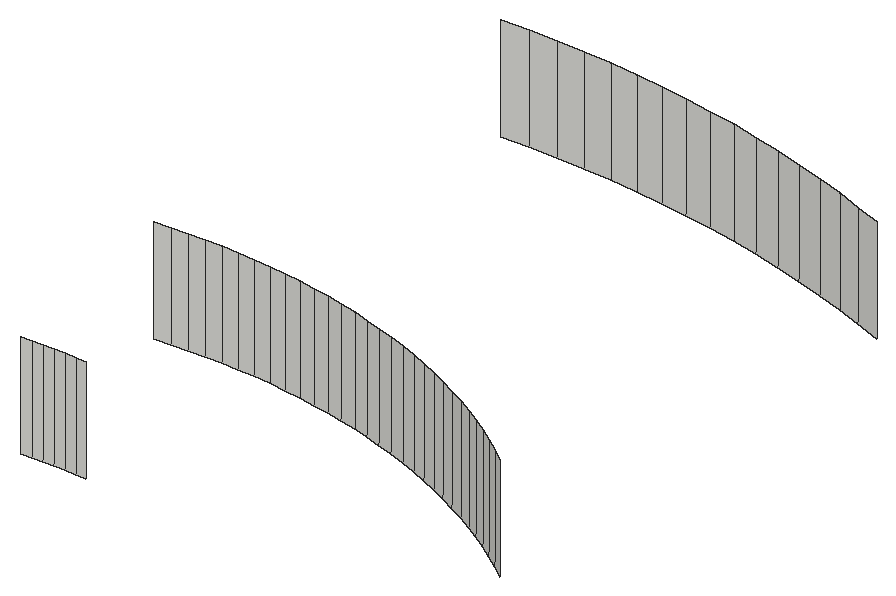
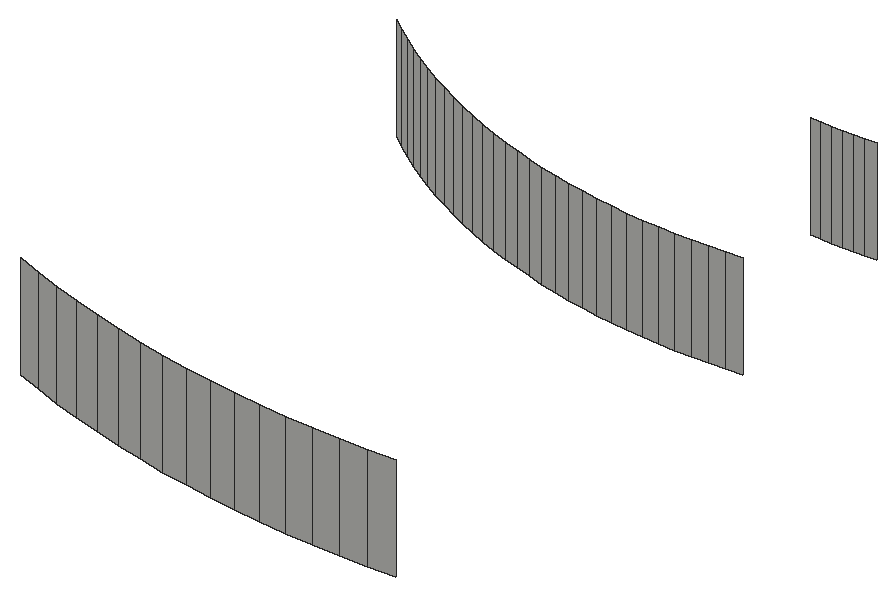
# SketchUp Ruby script. Lengths in inches.
U = 1.inch
M = Sketchup.active_model
def pt(a) = Geom::Point3d.new(a.map { |v| v * U })
def face(e, loops, mat)
  f = e.add_face(loops[0].map { |a| pt(a) })
  loops[1..].each { |l| e.add_face(l.map { |a| pt(a) }).erase! }
  f.material = f.back_material = mat if mat
  f
end
# faces: each face lists its corners as indices into pts; further lists are holes
def faces(e, pts, list, mat = nil) = list.each { |f| face(e, (f[0].is_a?(Array) ? f : [f]).map { |l| l.map { |i| pts[i] } }, mat) }
# xy, xz, yz: faces in a plane at the given z, y or x. An outline is a flat list of corners, or four numbers for a rectangle; further outlines are holes
def ring(l) = l.size == 4 ? [[l[0], l[1]], [l[2], l[1]], [l[2], l[3]], [l[0], l[3]]] : l.each_slice(2).to_a
def flat(e, list, mat, &to3) = list.each { |f| face(e, (f[0].is_a?(Array) ? f : [f]).map { |l| ring(l).map { |u, v| to3.(u, v) } }, mat) }
def xy(e, z, list, mat = nil) = flat(e, list, mat) { |x, y| [x, y, z] }
def xz(e, y, list, mat = nil) = flat(e, list, mat) { |x, z| [x, y, z] }
def yz(e, x, list, mat = nil) = flat(e, list, mat) { |y, z| [x, y, z] }
def lines(e, pts, list) = list.each { |a, b| e.add_line(pt(pts[a]), pt(pts[b])) }
# prism: a flat outline (further loops are holes) pulled along v
def prism(e, loops, v, mat = nil)
  f = face(e, loops, mat); d = Geom::Vector3d.new(v.map { |x| x * U })
  f.pushpull(f.normal.samedirection?(d) ? d.length : -d.length)
end
def box(e, o, s, mat = nil) = prism(e, [[o, [o[0] + s[0], o[1], o[2]], [o[0] + s[0], o[1] + s[1], o[2]], [o[0], o[1] + s[1], o[2]]]], [0, 0, s[2]], mat)
def at(x, y, z, deg = 0) = Geom::Transformation.translation(pt([x, y, z])) * Geom::Transformation.rotation(ORIGIN, Z_AXIS, deg.degrees)
def axes(o, x, y, z) = Geom::Transformation.new([*x, 0, *y, 0, *z, 0, *pt(o).to_a, 1])
def part(name) = M.definitions.add(name)
# library, detail: a bought-in or finely detailed component or shape, given as its bounding box
def library(name, o, s) = part(name).tap { |d| box(d.entities, o, s) }
def detail(e, o, s) = box(e.add_group.entities, o, s)
def put(e, d, t, mat = nil) = e.add_instance(d, t).tap { |i| i.material = mat if mat }
def group(e, t, mat = nil) = e.add_group.tap { |g| g.transformation = t; g.material = mat if mat }.entities
root = M.entities
p = [[904.72,349.22,117.3125],[904.1,349.18,117.3125],[904.1,349.18,111.3125],[904.72,349.22,111.3125],[905.35,349.25,117.3125],[905.35,349.25,111.3125],
  [905.98,349.26,117.3125],[905.98,349.26,111.3125],[906.61,349.25,117.3125],[906.61,349.25,111.3125],[907.23,349.22,117.3125],[907.23,349.22,111.3125],
  [907.86,349.18,117.3125],[907.86,349.18,111.3125],[927.14,354.38,117.3125],[927.89,353.82,117.3125],[927.89,353.82,111.3125],[927.14,354.38,111.3125],
  [926.37,354.92,117.3125],[926.37,354.92,111.3125],[925.59,355.45,117.3125],[925.59,355.45,111.3125],[924.79,355.95,117.3125],[924.79,355.95,111.3125],
  [923.98,356.43,117.3125],[923.98,356.43,111.3125],[923.16,356.89,117.3125],[923.16,356.89,111.3125],[922.32,357.33,117.3125],[922.32,357.33,111.3125],
  [921.48,357.75,117.3125],[921.48,357.75,111.3125],[920.62,358.14,117.3125],[920.62,358.14,111.3125],[919.76,358.52,117.3125],[919.76,358.52,111.3125],
  [918.88,358.87,117.3125],[918.88,358.87,111.3125],[918,359.19,117.3125],[918,359.19,111.3125],[917.1,359.49,117.3125],[917.1,359.49,111.3125],
  [916.2,359.77,117.3125],[916.2,359.77,111.3125],[915.3,360.03,117.3125],[915.3,360.03,111.3125],[914.38,360.26,117.3125],[914.38,360.26,111.3125],
  [913.46,360.47,117.3125],[913.46,360.47,111.3125],[912.54,360.65,117.3125],[912.54,360.65,111.3125],[911.61,360.8125,117.3125],[911.61,360.8125,111.3125],
  [910.68,360.95,117.3125],[910.68,360.95,111.3125],[909.74,361.06,117.3125],[909.74,361.06,111.3125],[902.22,361.06,117.3125],[903.15,361.15,117.3125],
  [903.15,361.15,111.3125],[902.22,361.06,111.3125],[904.09,361.21,117.3125],[904.09,361.21,111.3125],[907.86,361.21,117.3125],[908.8,361.15,117.3125],
  [908.8,361.15,111.3125],[907.86,361.21,111.3125],[905.04,361.24,117.3125],[905.04,361.24,111.3125],[905.98,361.26,117.3125],[905.98,361.26,111.3125],
  [906.92,361.24,117.3125],[906.92,361.24,111.3125],[927.48,381.27,117.3125],[926.01,381.81,117.3125],[926.01,381.81,111.3125],[927.48,381.27,111.3125],
  [924.52,382.32,117.3125],[924.52,382.32,111.3125],[923.02,382.79,117.3125],[923.02,382.79,111.3125],[921.51,383.21,117.3125],[921.51,383.21,111.3125],
  [919.99,383.6,117.3125],[919.99,383.6,111.3125],[918.45,383.95,117.3125],[918.45,383.95,111.3125],[916.91,384.25,117.3125],[916.91,384.25,111.3125],
  [915.36,384.52,117.3125],[915.36,384.52,111.3125],[913.81,384.74,117.3125],[913.81,384.74,111.3125],[912.25,384.93,117.3125],[912.25,384.93,111.3125],
  [910.6875,385.07,117.3125],[910.6875,385.07,111.3125],[909.12,385.17,117.3125],[909.12,385.17,111.3125],[904.41,385.24,117.3125],[902.84,385.17,117.3125],
  [902.84,385.17,111.3125],[904.41,385.24,111.3125],[905.98,385.26,117.3125],[905.98,385.26,111.3125],[907.55,385.24,117.3125],[907.55,385.24,111.3125]]
faces(root,p,[[0,1,2,3],[4,0,3,5],[6,4,5,7],[8,6,7,9],[10,8,9,11],[12,10,11,13],[14,15,16,17],[18,14,17,19],
  [20,18,19,21],[22,20,21,23],[24,22,23,25],[26,24,25,27],[28,26,27,29],[30,28,29,31],[32,30,31,33],[34,32,33,35],
  [36,34,35,37],[38,36,37,39],[40,38,39,41],[42,40,41,43],[44,42,43,45],[46,44,45,47],[48,46,47,49],[50,48,49,51],
  [52,50,51,53],[54,52,53,55],[56,54,55,57],[58,59,60,61],[59,62,63,60],[64,65,66,67],[65,56,57,66],[62,68,69,63],
  [68,70,71,69],[70,72,73,71],[72,64,67,73],[74,75,76,77],[75,78,79,76],[78,80,81,79],[80,82,83,81],[82,84,85,83],
  [84,86,87,85],[86,88,89,87],[88,90,91,89],[90,92,93,91],[92,94,95,93],[94,96,97,95],[96,98,99,97],[100,101,102,103],
  [104,100,103,105],[106,104,105,107],[98,106,107,99]])
